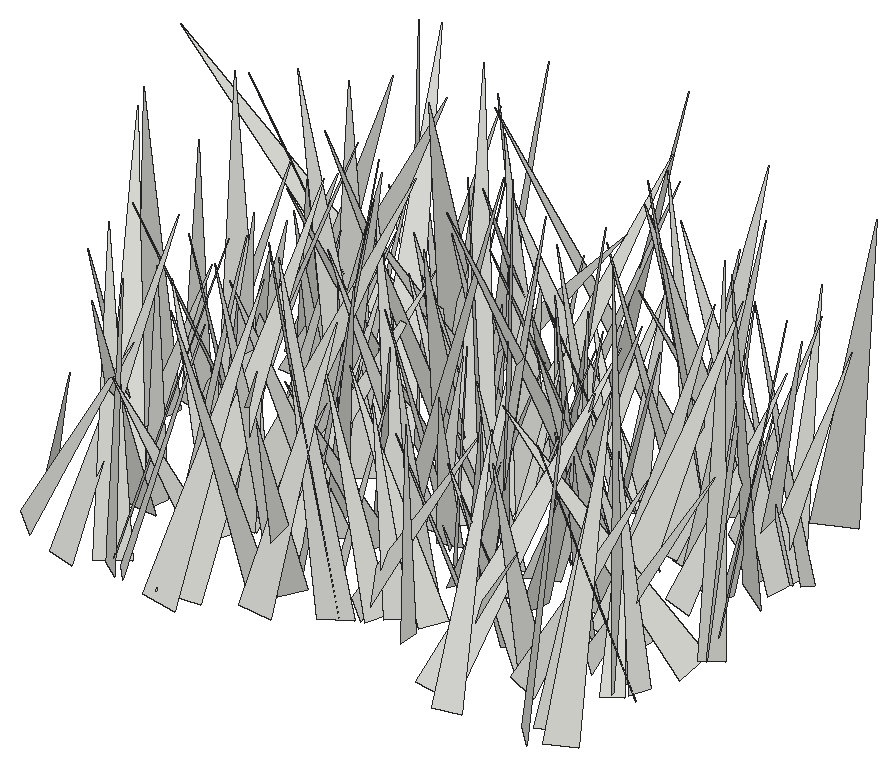
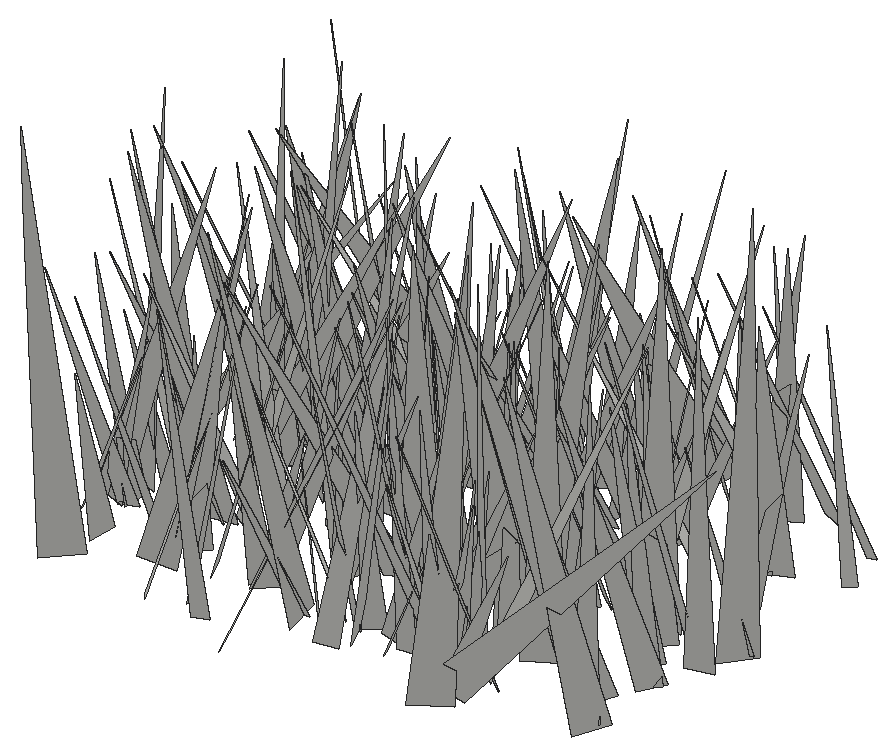
# SketchUp Ruby script. Lengths in inches.
U = 1.inch
M = Sketchup.active_model
def pt(a) = Geom::Point3d.new(a.map { |v| v * U })
def face(e, loops, mat)
  f = e.add_face(loops[0].map { |a| pt(a) })
  loops[1..].each { |l| e.add_face(l.map { |a| pt(a) }).erase! }
  f.material = f.back_material = mat if mat
  f
end
# faces: each face lists its corners as indices into pts; further lists are holes
def faces(e, pts, list, mat = nil) = list.each { |f| face(e, (f[0].is_a?(Array) ? f : [f]).map { |l| l.map { |i| pts[i] } }, mat) }
# xy, xz, yz: faces in a plane at the given z, y or x. An outline is a flat list of corners, or four numbers for a rectangle; further outlines are holes
def ring(l) = l.size == 4 ? [[l[0], l[1]], [l[2], l[1]], [l[2], l[3]], [l[0], l[3]]] : l.each_slice(2).to_a
def flat(e, list, mat, &to3) = list.each { |f| face(e, (f[0].is_a?(Array) ? f : [f]).map { |l| ring(l).map { |u, v| to3.(u, v) } }, mat) }
def xy(e, z, list, mat = nil) = flat(e, list, mat) { |x, y| [x, y, z] }
def xz(e, y, list, mat = nil) = flat(e, list, mat) { |x, z| [x, y, z] }
def yz(e, x, list, mat = nil) = flat(e, list, mat) { |y, z| [x, y, z] }
def lines(e, pts, list) = list.each { |a, b| e.add_line(pt(pts[a]), pt(pts[b])) }
# prism: a flat outline (further loops are holes) pulled along v
def prism(e, loops, v, mat = nil)
  f = face(e, loops, mat); d = Geom::Vector3d.new(v.map { |x| x * U })
  f.pushpull(f.normal.samedirection?(d) ? d.length : -d.length)
end
def box(e, o, s, mat = nil) = prism(e, [[o, [o[0] + s[0], o[1], o[2]], [o[0] + s[0], o[1] + s[1], o[2]], [o[0], o[1] + s[1], o[2]]]], [0, 0, s[2]], mat)
def at(x, y, z, deg = 0) = Geom::Transformation.translation(pt([x, y, z])) * Geom::Transformation.rotation(ORIGIN, Z_AXIS, deg.degrees)
def axes(o, x, y, z) = Geom::Transformation.new([*x, 0, *y, 0, *z, 0, *pt(o).to_a, 1])
def part(name) = M.definitions.add(name)
# library, detail: a bought-in or finely detailed component or shape, given as its bounding box
def library(name, o, s) = part(name).tap { |d| box(d.entities, o, s) }
def detail(e, o, s) = box(e.add_group.entities, o, s)
def put(e, d, t, mat = nil) = e.add_instance(d, t).tap { |i| i.material = mat if mat }
def group(e, t, mat = nil) = e.add_group.tap { |g| g.transformation = t; g.material = mat if mat }.entities
root = M.entities
c1 = part("fur_instance\#9")
p = [[0.8125,0,1.79],[0.67,-0.02,1.48],[0,-0.11,0],[0,0.11,0]]
faces(c1.entities,p,[[0,1,2,3]])
put(root,c1,axes([111.02,378.1875,-27.1],[4.54729,4.68314,2.12923],[4.88324,-4.82336,0.17985],[-1.61844,-1.39522,6.52513]))
put(root,c1,axes([92.14,378.47,-27.1],[3.06348,4.37723,2.06786],[4.6001,-3.39453,0.37061],[-1.50841,-1.46222,5.32989]))
put(root,c1,axes([97.12,380.5625,-27.1],[-5.96376,-1.66281,1.60864],[-1.32131,6.09893,1.40577],[1.89916,-0.97833,6.02952]))
put(root,c1,axes([98.24,381.11,-27.1],[3.42227,-3.49613,0.30492],[-3.40506,-3.41104,-0.89344],[-0.84941,-0.41195,4.81005]))
put(root,c1,axes([94.98,377.65,-27.1],[0.10942,6.44965,1.02032],[6.44115,0.06102,-1.07648],[1.07264,-1.02435,6.36012]))
put(root,c1,axes([87.73,379.19,-27.1],[2.82226,4.09729,0.68802],[3.94816,-2.38599,-1.98631],[1.29353,-1.65697,4.56152]))
put(root,c1,axes([107.76,377.89,-27.1],[-1.60174,4.9541,0.61833],[4.97114,1.64265,-0.28364],[0.46172,-0.4996,5.19887]))
put(root,c1,axes([87.05,381.24,-27.1],[4.69242,0.16576,0.10905],[0.19618,-4.2622,-1.96297],[-0.02968,-1.96577,4.26532]))
put(root,c1,axes([92.63,378.52,-27.1],[3.7464,3.46532,0.67043],[3.46985,-3.79505,0.22613],[-0.64655,-0.28736,5.09832]))
put(root,c1,axes([91.81,379,-27.1],[-3.36286,5.21282,1.50099],[5.38655,3.41774,0.19865],[0.64152,-1.37145,6.20023]))
put(root,c1,axes([105.42,380.92,-27.1],[3.7363,2.07589,0.22504],[1.88074,-3.14536,-2.2112],[0.90706,-2.02911,3.65784]))
put(root,c1,axes([90.27,382.49,-27.1],[0.60186,-6.09784,0.10298],[-6.0697,-0.58883,0.60707],[0.59415,0.16161,6.09732]))
put(root,c1,axes([93.92,381.71,-27.1],[-4.12735,0.23871,1.0618],[0.66209,3.85593,1.70672],[0.86374,-1.81501,3.76552]))
put(root,c1,axes([98.04,379.23,-27.1],[-0.68675,5.73435,1.62653],[5.78722,1.03346,-1.2],[1.42703,-1.4315,5.64928]))
put(root,c1,axes([108.55,381.74,-27.1],[4.51587,-1.82573,1.61231],[-1.49442,-4.75873,-1.20297],[-1.92343,-0.58918,4.72009]))
put(root,c1,axes([90.3125,377.95,-27.1],[2.22729,6.28936,0.04999],[6.2767,-2.22605,0.40869],[-0.40191,0.08939,6.65956]))
put(root,c1,axes([100.12,381.12,-27.1],[4.02018,4.80904,4.066],[5.52928,-5.00439,0.45193],[-3.01434,-2.76593,6.25176]))
put(root,c1,axes([94.29,379.04,-27.1],[4.06792,5.19434,1.22411],[5.14399,-4.22635,0.83955],[-1.42088,-0.42943,6.54403]))
put(root,c1,axes([100.61,380.57,-27.1],[0.55965,-6.1533,3.26603],[-6.71098,-1.35523,-1.40332],[-1.86889,3.02383,6.01722]))
put(root,c1,axes([112.45,378.46,-27.1],[-5.42402,3.35952,0.54018],[3.08821,5.28712,-1.87283],[1.42868,1.32596,6.09909]))
put(root,c1,axes([106.79,382.85,-27.1],[1.2889,-4.23263,0.01136],[-4.22076,-1.28617,-0.32791],[-0.31699,-0.08469,4.41236]))
put(root,c1,axes([111.32,379.04,-27.1],[-4.3486,2.21974,0.80785],[1.83051,4.23636,-1.78683],[1.49303,1.27131,4.54366]))
put(root,c1,axes([103.45,381.11,-27.1],[-3.94466,-0.14605,1.57067],[-0.23954,4.23653,-0.20765],[1.55915,0.28136,3.94189]))
put(root,c1,axes([111.99,383.04,-27.1],[-3.65311,-4.50937,0.62916],[-4.48426,3.70309,0.50402],[0.78847,0.16789,5.78149]))
put(root,c1,axes([108.77,380.85,-27.1],[0.87918,5.14411,1.43079],[4.85097,-0.16366,-2.39235],[2.23095,-1.67133,4.63805]))
put(root,c1,axes([108.61,381.42,-27.1],[-0.27177,-3.75184,1.87256],[-3.70908,-0.66019,-1.86105],[-1.95589,1.77327,3.26904]))
put(root,c1,axes([96.52,382.55,-27.1],[-6.02473,-0.71032,1.74625],[-0.51818,6.24626,0.75302],[1.81257,-0.57532,6.01954]))
put(root,c1,axes([101.71,381.58,-27.1],[-4.44101,1.77663,0.66677],[1.83519,4.45274,0.3588],[0.48276,-0.58331,4.76973]))
put(root,c1,axes([106.6,378.69,-27.1],[-2.65177,6.66161,0.65253],[5.97681,2.67255,-2.995],[3.01341,0.56142,6.51452]))
put(root,c1,axes([100.72,381.58,-27.1],[2.95433,4.07724,0.35212],[3.82019,-2.59183,-2.04072],[1.46767,-1.46099,4.60298]))
put(root,c1,axes([93.55,382.24,-27.1],[4.21997,-0.6182,0.41958],[-0.60999,-4.24047,-0.11271],[-0.43142,-0.05127,4.26352]))
put(root,c1,axes([104.69,382.98,-27.1],[5.27182,0.13194,1.25121],[0.40362,-5.28245,-1.14356],[-1.19165,-1.2055,5.14798]))
put(root,c1,axes([95.3,378.33,-27.1],[-5.76444,5.45156,1.05869],[4.71185,5.60881,-3.22628],[2.93919,1.70025,7.24841]))
put(root,c1,axes([102.25,381.94,-27.1],[-2.34318,3.21724,1.23905],[3.43189,2.31946,0.46753],[0.3286,-1.2829,3.95253]))
put(root,c1,axes([91.68,379.35,-27.1],[4.88269,3.53574,0.69101],[3.04894,-4.67553,2.3797],[-1.91908,1.56767,5.53887]))
put(root,c1,axes([103.54,382.43,-27.1],[-3.16425,3.77948,0.90882],[3.82647,2.82214,1.58634],[-0.68447,-1.69527,4.66695]))
put(root,c1,axes([90.54,383.03,-27.1],[4.66089,-0.94094,1.87831],[-0.93791,-5.02216,-0.1885],[-1.87983,0.17273,4.75118]))
put(root,c1,axes([99.8,381.32,-27.1],[2.15657,3.40289,0.33157],[3.29952,-2.17412,0.8525],[-0.89598,0.18416,3.93747]))
put(root,c1,axes([93.79,382.68,-27.1],[-4.37438,2.14658,0.79892],[2.22863,4.38643,0.41683],[0.52851,-0.72986,4.85482]))
put(root,c1,axes([106.63,379.97,-27.1],[4.76717,4.34009,0.09976],[4.0907,-4.54047,2.05487],[-1.45344,1.45601,6.11063]))
put(root,c1,axes([104.82,383.17,-27.1],[-3.19994,-2.12817,0.10035],[-2.08753,3.09569,-0.91527],[-0.42587,0.81635,3.73243]))
put(root,c1,axes([94.13,383.44,-27.1],[2.50338,-2.82714,1.30611],[-3.05988,-2.54469,0.35667],[-0.57944,1.22368,3.75931]))
put(root,c1,axes([89.07,384.27,-27.1],[-1.67954,-4.60165,1.09216],[-4.72861,1.65608,-0.29411],[0.09072,1.12742,4.88974]))
put(root,c1,axes([93.97,384.37,-27.1],[-1.02707,-3.52995,0.46815],[-3.49734,0.90838,-0.82343],[-0.66956,0.66999,3.58293]))
put(root,c1,axes([101.92,383.99,-27.1],[0.28904,-4.61969,1.68996],[-4.89331,-0.44312,-0.3744],[-0.50298,1.65624,4.61355]))
put(root,c1,axes([111.68,382.29,-27.1],[-2.57238,2.98987,0.10946],[2.97729,2.57237,-0.29516],[0.29502,0.10983,3.93311]))
put(root,c1,axes([98.65,385.7,-27.1],[1.56687,-4.2825,0.24372],[-4.04586,-1.5617,-1.43053],[-1.42486,-0.27491,4.32996]))
put(root,c1,axes([112.21,383.17,-27.1],[-4.36363,0.98227,0.81119],[0.91976,4.432,-0.41906],[0.88144,0.23814,4.45315]))
put(root,c1,axes([97.375,382.64,-27.1],[5.30824,4.83924,1.79848],[4.88732,-5.54151,0.48577],[-1.6634,-0.83881,7.16657]))
put(root,c1,axes([97.09,385.17,-27.1],[0.61294,-5.47928,1.38132],[-5.30961,-1.0339,-1.7451],[-1.93355,1.10218,5.22999]))
put(root,c1,axes([112.61,385.73,-27.1],[-5.96221,1.49508,0.02596],[1.36332,5.39133,2.61894],[-0.61423,-2.54602,5.56097]))
put(root,c1,axes([109.48,383.72,-27.1],[3.29682,4.04593,0.27696],[3.82738,-2.98619,-1.93627],[1.34069,-1.42422,4.84659]))
put(root,c1,axes([111.5,383.03,-27.1],[-7.33304,-1.55705,2.53328],[-2.07568,7.50758,-1.39398],[2.1292,1.95633,7.36578]))
put(root,c1,axes([107.93,385.49,-27.1],[-3.27673,-6.38483,2.25273],[-6.55108,3.62196,0.73666],[1.71005,1.64109,7.13865]))
put(root,c1,axes([96.43,385.79,-27.1],[6.1777,-0.38175,1.16241],[-0.13775,-6.16226,-1.29169],[-1.21571,-1.24165,6.0532]))
put(root,c1,axes([108.61,386.8125,-27.1],[1.25653,-6.81976,0.6894],[-6.81087,-1.32116,-0.65555],[-0.77223,0.55558,6.90349]))
put(root,c1,axes([89.71,382.25,-27.1],[-3.35316,6.39569,0.22234],[6.39729,3.34326,0.30873],[-0.17041,-0.34016,7.2148]))
put(root,c1,axes([92.72,385.62,-27.1],[-4.52954,-3.25843,1.35312],[-3.24257,4.71245,0.49358],[1.39071,0.3748,5.55792]))
put(root,c1,axes([90.9,388.14,-27.1],[-3.5223,-6.70382,0.02091],[-6.50166,3.42181,1.83516],[1.63401,-0.83562,7.34711]))
put(root,c1,axes([105.59,385.52,-27.1],[5.75538,-1.33671,0.29214],[-1.31847,-5.75568,-0.36093],[-0.36579,-0.28603,5.89753]))
put(root,c1,axes([96.39,383.14,-27.1],[-0.08905,4.06249,0.07241],[4.03019,0.09752,-0.5148],[0.51634,-0.06053,4.03072]))
put(root,c1,axes([96.22,384.53,-27.1],[6.38411,4.40631,2.11358],[4.61615,-6.57865,-0.22824],[-1.60436,-1.39477,7.75373]))
put(root,c1,axes([97.61,386.74,-27.1],[4.97524,0.71585,1.07536],[1.04452,-4.74693,-1.67259],[-0.76015,-1.83742,4.74004]))
put(root,c1,axes([110.31,386.29,-27.1],[-3.89042,0.9571,1.21715],[1.27935,3.84105,1.06884],[0.87221,-1.36496,3.86121]))
put(root,c1,axes([93.42,384.34,-27.1],[2.59444,7.48207,1.23534],[7.31718,-2.12705,-2.48457],[1.99156,-1.93206,7.51927]))
put(root,c1,axes([100.42,387.22,-27.1],[1.67975,-3.93598,0.16611],[-3.93538,-1.66827,0.26597],[0.17974,0.25696,4.27115]))
put(root,c1,axes([100.32,384.88,-27.1],[-1.21025,6.4146,1.42422],[6.45546,0.89059,1.47445],[-1.22575,-1.64315,6.35907]))
put(root,c1,axes([86.81,387.85,-27.1],[7.55718,-3.05255,1.8054],[-2.7949,-7.74218,-1.39129],[-2.18313,-0.65505,8.03077]))
put(root,c1,axes([91.96,383.52,-27.1],[5.80303,5.01805,0.27093],[4.96083,-5.78629,0.91567],[-0.80277,0.51711,7.61693]))
put(root,c1,axes([107.73,386.65,-27.1],[0.85171,-3.4207,0.8533],[-3.50883,-0.73716,0.54719],[0.34265,0.95401,3.48241]))
put(root,c1,axes([101.58,386.0625,-27.1],[3.14318,2.78213,1.66083],[2.96777,-3.40061,0.07991],[-1.30037,-1.03624,4.19683]))
put(root,c1,axes([103.09,385.67,-27.1],[4.37398,5.97616,2.1686],[6.29129,-4.44766,-0.43255],[-0.91492,-2.01317,7.39318]))
put(root,c1,axes([102.34,385.09,-27.1],[4.56042,0.58445,0.815],[0.35248,-4.48653,1.24501],[-0.93891,1.15443,4.42595]))
put(root,c1,axes([100.34,387.48,-27.1],[-4.23671,-2.59002,0.97553],[-2.55905,4.34534,0.42292],[1.0541,0.13924,4.94763]))
put(root,c1,axes([104.03,385.76,-27.1],[-6.60957,-3.13791,3.29203],[-3.79035,7.01015,-0.92809],[2.51341,2.31982,7.25752]))
put(root,c1,axes([98.69,388.15,-27.1],[-5.81258,-1.56867,1.18702],[-1.32265,5.85738,1.26392],[1.45614,-0.94136,5.88637]))
put(root,c1,axes([100.27,384.14,-27.1],[7.12046,1.58475,2.39098],[0.70942,-7.17277,2.64146],[-2.77938,2.22916,6.79964]))
put(root,c1,axes([103.33,387.27,-27.1],[-0.82021,3.34867,1.94688],[3.86928,0.61559,0.57127],[-0.18046,-2.02092,3.4]))
put(root,c1,axes([108.05,388.35,-27.1],[-2.49506,-7.82927,1.12782],[-7.54738,2.00233,-2.79687],[-2.3678,1.86761,7.7266]))
put(root,c1,axes([94.34,385.67,-27.1],[1.81357,5.35205,0.20733],[5.12174,-1.66889,-1.72019],[1.56691,-0.73948,5.38279]))
put(root,c1,axes([93.54,388.57,-27.1],[5.39011,-5.98506,0.75501],[-6.02641,-5.29691,1.03406],[0.27067,1.25142,7.9878]))
put(root,c1,axes([108.91,385.56,-27.1],[-0.63507,6.95916,1.46669],[6.78735,1.03289,-1.962],[2.12438,-1.21968,6.70699]))
put(root,c1,axes([104.47,387.36,-27.1],[5.13759,-3.83835,0.8309],[-3.9202,-4.93031,1.46363],[0.23526,1.66651,6.24384]))
put(root,c1,axes([104.13,385.58,-27.1],[0.66695,4.37993,0.08385],[4.36286,-0.67176,0.3871],[-0.39533,-0.02429,4.41347]))
put(root,c1,axes([95.62,387.45,-27.1],[-2.49049,-3.07283,1.62396],[-3.33154,2.67981,-0.03854],[0.99012,1.28779,3.95516]))
put(root,c1,axes([89.54,388.18,-27.1],[3.73813,0.01426,0.67221],[0.17612,-3.68545,-0.90117],[-0.64889,-0.91811,3.62791]))
put(root,c1,axes([86.79,387.37,-27.1],[-0.2038,-3.57727,1.86557],[-3.68837,0.92217,1.36537],[1.63497,1.63446,3.31273]))
put(root,c1,axes([99.51,387.64,-27.1],[1.31397,-3.56018,1.31098],[-3.78942,-1.16427,0.63629],[0.18405,1.44556,3.7412]))
put(root,c1,axes([108.75,388.19,-27.1],[-4.44374,-5.75342,0.61079],[-5.6055,4.0905,-2.25122],[-1.43294,1.84058,6.91236]))
put(root,c1,axes([94.58,388.18,-27.1],[3.50873,2.55931,1.93983],[3.03472,-3.58228,-0.76287],[-1.05048,-1.80039,4.27543]))
put(root,c1,axes([89.55,388.72,-27.1],[3.84963,-3.94903,0.87916],[-4.01863,-3.87266,0.20133],[-0.4673,0.77142,5.51126]))
put(root,c1,axes([90.29,388.09,-27.1],[4.03772,-5.94106,3.0996],[-6.44975,-4.42725,-0.08397],[-1.8178,2.512,7.18278]))
put(root,c1,axes([98.27,390.36,-27.1],[2.21636,-6.61774,0.25451],[-6.61771,-2.20273,0.35418],[0.25535,0.35358,6.97003]))
put(root,c1,axes([104.12,389.3,-27.1],[-2.04339,-2.88899,0.9747],[-2.5158,2.26047,1.42575],[1.7225,-0.12566,3.23866]))
put(root,c1,axes([102.68,385.76,-27.1],[-0.48607,6.36101,0.33267],[6.36907,0.48063,0.1158],[-0.09028,-0.34048,6.37851]))
put(root,c1,axes([87.42,389.26,-27.1],[0.11264,-6.37998,1.60761],[-6.5012,0.13924,1.0081],[1.01142,1.60553,6.30084]))
put(root,c1,axes([99.97,389.51,-27.1],[-2.55131,-7.67351,1.38924],[-7.65133,2.18082,-2.00574],[-1.50657,1.91917,7.83383]))
put(root,c1,axes([92.95,387.48,-27.1],[3.70587,4.25797,0.60198],[4.28884,-3.60158,-0.92773],[0.31394,-1.06043,5.56805]))
put(root,c1,axes([105.88,387.66,-27.1],[2.53366,4.26731,1.78001],[4.34271,-2.89305,0.75426],[-1.5872,-1.10369,4.90515]))
put(root,c1,axes([92.89,386.33,-27.1],[-4.41851,1.16155,1.66424],[0.34777,4.36157,-2.12081],[1.99949,1.8082,4.04655]))
put(root,c1,axes([106.66,391.01,-27.1],[-4.09518,-5.32392,0.52178],[-5.17841,4.11019,1.29512],[1.34181,-0.38619,6.5907]))
put(root,c1,axes([94.41,387.38,-27.1],[1.13394,4.06883,0.24777],[4.07369,-1.14042,0.08414],[-0.14769,-0.216,4.22305]))
put(root,c1,axes([88.21,388.52,-27.1],[3.54049,4.95211,1.34575],[5.12044,-3.30078,-1.32493],[0.33991,-1.85767,5.94164]))
put(root,c1,axes([104.58,391.06,-27.1],[6.71484,1.18998,0.43364],[1.2609,-6.06064,-2.89345],[0.11927,-2.92333,6.1752]))
put(root,c1,axes([101.95,387.3,-27.1],[-6.04222,-2.58238,2.07365],[-3.21518,5.60869,-2.38377],[0.79453,3.05796,6.1233]))
put(root,c1,axes([94.92,389.0625,-27.1],[1.79805,-6.87497,3.712],[-7.43664,-2.674,-1.35027],[-2.39594,3.14033,6.97674]))
put(root,c1,axes([112.47,386.4,-27.1],[3.51213,5.3509,1.08193],[4.75447,-3.63032,2.52063],[-2.68285,0.57134,5.88334]))
put(root,c1,axes([107.41,388.23,-27.1],[1.23681,5.98503,1.54047],[6.1022,-0.934,-1.27052],[0.97821,-1.7408,5.97797]))
put(root,c1,axes([112.8,386.5,-27.1],[-7.06937,0.92542,0.80535],[0.55425,6.6114,-2.73188],[1.09444,2.62944,6.58553]))
put(root,c1,axes([88.97,390.03,-27.1],[3.21186,-3.52218,0.8528],[-3.62385,-3.13,0.72104],[-0.02677,1.11644,4.71189]))
put(root,c1,axes([88.02,391.3,-27.1],[0.93957,-4.99379,0.05949],[-4.70596,-0.86502,1.71172],[1.67197,0.37157,4.78443]))
put(root,c1,axes([96.04,391.78,-27.1],[-1.10699,-6.38687,0.31821],[-6.26084,1.01671,-1.37367],[-1.30201,0.54128,6.33487]))
put(root,c1,axes([111.6875,388.42,-27.1],[-4.45958,-2.36263,3.46386],[-3.3219,5.07642,-0.81428],[2.55838,2.47306,4.98064]))
put(root,c1,axes([111.05,390.96,-27.1],[-3.13728,-6.42445,2.27927],[-6.51063,3.56742,1.09378],[2.01998,1.52023,7.06539]))
put(root,c1,axes([99.96,389.21,-27.1],[-1.66543,4.2087,0.7623],[4.0491,1.28782,1.73616],[-1.37806,-1.30242,4.18002]))
put(root,c1,axes([94.3,391.71,-27.1],[-0.53016,-5.209,0.61736],[-4.97847,0.69512,1.58982],[1.65216,0.4231,4.98871]))
put(root,c1,axes([109.42,388.78,-27.1],[0.30593,5.01742,0.69432],[4.86404,-0.09691,-1.44288],[1.4134,-0.75252,4.8152]))
put(root,c1,axes([91.51,391.4,-27.1],[4.6906,-0.13116,1.94102],[0.35682,-4.92253,-1.19491],[-1.91244,-1.24013,4.53774]))
put(root,c1,axes([93.81,391.98,-27.1],[5.31663,-1.02418,0.76649],[-0.77202,-5.18142,-1.56841],[-1.02002,-1.41668,5.18224]))
put(root,c1,axes([102.05,391.25,-27.1],[6.71325,2.37054,1.67819],[2.73448,-6.58312,-1.63968],[-0.97898,-2.13225,6.9281]))
put(root,c1,axes([97.625,391.22,-27.1],[3.16597,-2.82128,1.36449],[-2.73379,-3.43456,-0.75836],[-1.53229,0.2984,4.17228]))
put(root,c1,axes([98.09,391.84,-27.1],[2.45481,-4.16097,0.8917],[-4.06011,-2.59844,-0.9479],[-1.27449,0.26329,4.73722]))
put(root,c1,axes([110.41,390.35,-27.1],[3.57631,0.31891,0.97988],[0.16002,-3.66803,0.60973],[-1.01797,0.54376,3.53835]))
put(root,c1,axes([97.04,392.58,-27.1],[-3.71631,2.59474,2.95715],[3.6126,3.86147,1.15179],[1.55775,-2.76492,4.38373]))
put(root,c1,axes([100.15,388.98,-27.1],[-7.18499,4.19207,1.05141],[4.04317,7.24035,-1.23823],[1.52698,0.55406,8.22584]))
put(root,c1,axes([101,391.35,-27.1],[-6.55699,2.55506,2.62376],[2.8465,6.94107,0.35432],[2.30431,-1.30376,7.02829]))
put(root,c1,axes([108.68,390.63,-27.1],[3.30058,6.51639,2.13105],[6.85171,-3.21879,-0.76942],[-0.24255,-2.25268,7.26396]))
put(root,c1,axes([92.1,392.19,-27.1],[3.60415,-6.43604,2.10161],[-6.7075,-3.71823,0.11619],[-0.92131,1.89247,7.37557]))
put(root,c1,axes([104.625,390.7,-27.1],[-5.51822,-0.21879,0.79161],[-0.32668,5.51842,-0.75206],[0.75352,0.79022,5.4711]))
put(root,c1,axes([87.93,391.28,-27.1],[2.95683,-4.48742,1.40063],[-4.613,-2.45121,1.88504],[0.90496,2.16707,5.03253]))
put(root,c1,axes([96.84,395.17,-27.1],[-5.64756,-4.03637,0.24701],[-3.60758,5.22048,2.82493],[1.82721,-2.16853,6.3409]))
put(root,c1,axes([111.53,392.29,-27.1],[-7.04891,1.70289,1.4017],[1.92518,7.04086,1.12767],[1.07622,-1.44158,7.16347]))
put(root,c1,axes([102.21,391.21,-27.1],[-3.53666,-0.44387,1.07965],[-0.6619,3.59984,-0.68824],[0.96154,0.84544,3.49732]))
put(root,c1,axes([92.99,390.71,-27.1],[2.64907,4.14771,0.84835],[4.17625,-2.72433,0.27885],[-0.69438,-0.56151,4.91358]))
put(root,c1,axes([101.12,392.3,-27.1],[-2.05485,-3.90462,0.97999],[-3.96047,1.76344,-1.27819],[-0.72186,1.43981,4.22312]))
put(root,c1,axes([96.21,392.63,-27.1],[-2.14589,-4.13922,0.79032],[-4.13009,1.88974,-1.31675],[-0.83673,1.28775,4.4726]))
put(root,c1,axes([98.83,396.02,-27.1],[-2.64275,-7.72517,0.10148],[-7.35563,2.5487,2.46402],[2.36287,-0.70608,7.78402]))
put(root,c1,axes([93.26,393.9,-27.1],[-4.92734,-5.46841,0.2776],[-5.45988,4.87887,-0.80338],[-0.41255,0.74316,7.31688]))
put(root,c1,axes([111.28,392.46,-27.1],[-0.94166,-4.10224,1.61468],[-4.38512,0.70145,-0.77524],[-0.45421,1.73259,4.13692]))
put(root,c1,axes([108.26,392.5,-27.1],[-6.28358,-3.49392,1.76213],[-3.72095,6.36668,-0.64478],[1.21124,1.43309,7.16066]))
put(root,c1,axes([110.57,392.06,-27.1],[4.80103,-0.44543,1.50068],[-0.59366,-4.99749,0.41591],[-1.44845,0.57184,4.80368]))
put(root,c1,axes([88.14,394.76,-27.1],[0.06322,-6.05576,0.15688],[-5.74231,-0.00994,1.93043],[1.92942,0.16885,5.74018]))
put(root,c1,axes([106.89,390.25,-27.1],[5.00084,3.55671,0.83126],[3.26277,-4.98345,1.69387],[-1.6418,0.92989,5.89825]))
put(root,c1,axes([95.6,389.62,-27.1],[-4.43994,6.98412,0.3729],[6.94517,4.45476,-0.74146],[0.82561,0.08476,8.24265]))
put(root,c1,axes([106.48,393.44,-27.1],[3.38817,-1.89067,0.4047],[-1.85762,-3.4096,-0.37677],[-0.53632,-0.13453,3.86165]))
put(root,c1,axes([107.46,391.28,-27.1],[1.47589,3.3854,0.35503],[3.34161,-1.51469,0.55196],[-0.64858,-0.1002,3.65165]))
put(root,c1,axes([107.42,391.35,-27.1],[0.16612,7.76506,1.97129],[7.95416,0.07536,-0.96713],[0.95574,-1.97685,7.70638]))
put(root,c1,axes([99.72,394.08,-27.1],[-3.13954,-2.86345,1.03549],[-2.74612,3.30524,0.81394],[1.31545,0.06589,4.17056]))
put(root,c1,axes([88.87,393.33,-27.1],[4.47531,-6.51665,1.20055],[-6.35255,-3.80729,3.0143],[1.88498,2.64087,7.30815]))
put(root,c1,axes([103.07,394.12,-27.1],[-6.35837,1.48,1.02188],[1.69793,6.17763,1.61781],[0.593,-1.81932,6.3247]))
put(root,c1,axes([96.82,392.96,-27.1],[3.38987,-1.12165,1.00676],[-1.27426,-3.45624,0.43994],[-0.80492,0.7478,3.54341]))
put(root,c1,axes([110.53,392.5,-27.1],[0.61438,4.77457,1.24038],[4.786,-0.27399,-1.3159],[1.1955,-1.35681,4.63059]))
put(root,c1,axes([99.86,390.54,-27.1],[0.36828,7.38641,0.21711],[7.15433,-0.30198,-1.86176],[1.84979,-0.30261,7.15741]))
put(root,c1,axes([96.3125,394.59,-27.1],[-1.36067,-5.7583,1.83351],[-5.61411,1.9,1.80082],[2.23642,1.26617,5.63617]))
put(root,c1,axes([103.92,392.9375,-27.1],[-2.71204,2.5664,0.21286],[2.56651,2.66825,0.52947],[-0.21147,-0.53003,3.69611]))
put(root,c1,axes([107.15,395.15,-27.1],[1.49882,-6.76146,1.59023],[-6.75855,-1.79498,-1.262],[-1.60255,1.24632,6.80963]))
put(root,c1,axes([100.41,394.47,-27.1],[3.23905,1.92957,1.10614],[2.22288,-2.8741,-1.49551],[-0.07469,-1.85863,3.46094]))
put(root,c1,axes([98.2,394.05,-27.1],[2.26375,-3.28304,0.92587],[-3.40814,-2.22313,0.4499],[-0.14199,1.01955,3.96238]))
put(root,c1,axes([97.3125,394.24,-27.1],[-0.77658,-4.10323,1.17838],[-4.23531,0.59015,-0.73621],[-0.53592,1.28194,4.11067]))
put(root,c1,axes([105.3,394.21,-27.1],[-4.90258,-2.23132,0.87524],[-2.28191,4.95484,-0.15015],[0.73329,0.50088,5.38438]))
put(root,c1,axes([107.61,392.51,-27.1],[-6.80477,1.06742,0.77743],[0.9228,6.76292,-1.20833],[0.94457,1.0827,6.78117]))
put(root,c1,axes([94.0625,395.1,-27.1],[5.26826,5.58359,0.80335],[4.69893,-3.73546,-4.8521],[3.1212,-3.80083,5.9488]))
put(root,c1,axes([93.42,393.96,-27.1],[4.5767,5.68819,3.18986],[6.17982,-5.02762,0.09872],[-2.08339,-2.41752,7.30013]))
put(root,c1,axes([103.42,393.82,-27.1],[3.51253,-2.51047,1.78394],[-2.89575,-3.6135,0.61652],[-1.0486,1.56939,4.2732]))
put(root,c1,axes([93.25,397.12,-27.1],[6.31463,-5.10403,0.36931],[-4.97216,-6.25818,-1.47472],[-1.21044,-0.91981,7.98441]))
put(root,c1,axes([93.05,395.46,-27.1],[3.48904,-1.79502,0.75996],[-1.60226,-3.52839,-0.97792],[-1.11014,-0.54905,3.7999]))
put(root,c1,axes([112.08,392.82,-27.1],[-5.07583,-0.99149,0.0646],[-0.93064,4.62637,-2.11704],[-0.34804,2.08923,4.7186]))
put(root,c1,axes([98.78,394.3125,-27.1],[2.69077,3.3772,1.27263],[3.60609,-2.57991,-0.77814],[-0.14558,-1.48455,4.24737]))
put(root,c1,axes([108.22,393.57,-27.1],[2.30047,4.4169,0.81433],[4.47004,-2.16262,-0.89782],[0.43686,-1.13065,4.89848]))
put(root,c1,axes([106,397.24,-27.1],[-4.51609,-3.87484,0.43498],[-3.47065,4.29803,2.25393],[1.77713,-1.453,5.5072]))
put(root,c1,axes([97.33,392.75,-27.1],[4.31579,6.0344,1.65644],[5.97789,-4.5707,1.07586],[-1.85004,-0.69181,7.34048]))
put(root,c1,axes([93.36,395.49,-27.1],[0.28978,-3.77503,0.68612],[-3.83038,-0.24462,0.27184],[0.22308,0.70349,3.77636]))
put(root,c1,axes([98.49,394.71,-27.1],[5.38161,2.47127,3.67462],[2.66712,-6.4254,0.41515],[-3.53503,-1.08568,5.90733]))
put(root,c1,axes([87.71,394.95,-27.1],[5.60342,-3.67276,1.04707],[-3.81273,-5.48708,1.15708],[-0.22057,1.54484,6.59914]))
put(root,c1,axes([99.76,393.83,-27.1],[4.90909,4.36789,0.50992],[4.39704,-4.86378,-0.66882],[0.06695,-0.83837,6.53684]))
put(root,c1,axes([95.2,393.79,-27.1],[-4.58169,-0.00231,0.33908],[-0.10273,4.38765,-1.35823],[0.32316,1.36211,4.37574]))
put(root,c1,axes([93.56,395.93,-27.1],[-5.86481,5.71927,0.12396],[4.62698,4.63811,4.91939],[-3.36399,-3.59156,6.55024]))
put(root,c1,axes([104.71,396.29,-27.1],[4.53456,1.85789,3.16607],[2.55783,-5.20835,-0.60709],[-2.63311,-1.85992,4.86266]))
put(root,c1,axes([93.76,395.97,-27.1],[0.23103,-4.99246,1.62863],[-5.17408,0.0623,0.92493],[0.89778,1.64376,4.91147]))
put(root,c1,axes([110.09,396.79,-27.1],[4.60789,-6.31495,1.14074],[-6.41656,-4.51508,0.92427],[0.08686,1.46561,7.76253]))
put(root,c1,axes([100.75,394.98,-27.1],[7.58691,1.58366,1.76713],[1.48707,-7.78642,0.59349],[-1.84915,0.23586,7.72768]))
put(root,c1,axes([93.61,395.45,-27.1],[-2.38468,3.13652,0.12042],[3.02513,2.25628,1.13874],[-0.83714,-0.7813,3.77197]))
put(root,c1,axes([101.76,398.11,-27.1],[-6.74137,-3.47517,0.05647],[-3.44773,6.70195,0.85032],[0.43951,-0.73012,7.53656]))
put(root,c1,axes([92.57,394.4,-27.1],[3.35621,4.76804,0.53975],[4.75729,-3.3924,0.38655],[-0.62744,-0.21695,5.81798]))
put(root,c1,axes([100.91,394.81,-27.1],[0.42201,3.83383,0.13948],[3.79822,-0.3978,-0.55775],[0.53966,-0.19825,3.81644]))
put(root,c1,axes([94.56,394.65,-27.1],[3.67967,2.76321,1.03507],[2.46473,-3.78797,1.35021],[-1.62229,0.51247,4.39911]))
put(root,c1,axes([103.48,397.28,-27.1],[-0.9776,-5.25666,1.94415],[-5.10339,1.65068,1.89699],[2.31681,1.41798,4.99896]))
put(root,c1,axes([109.98,394.68,-27.1],[-4.30895,1.90574,0.59057],[1.67064,4.21479,-1.41144],[1.09067,1.07302,4.49519]))
